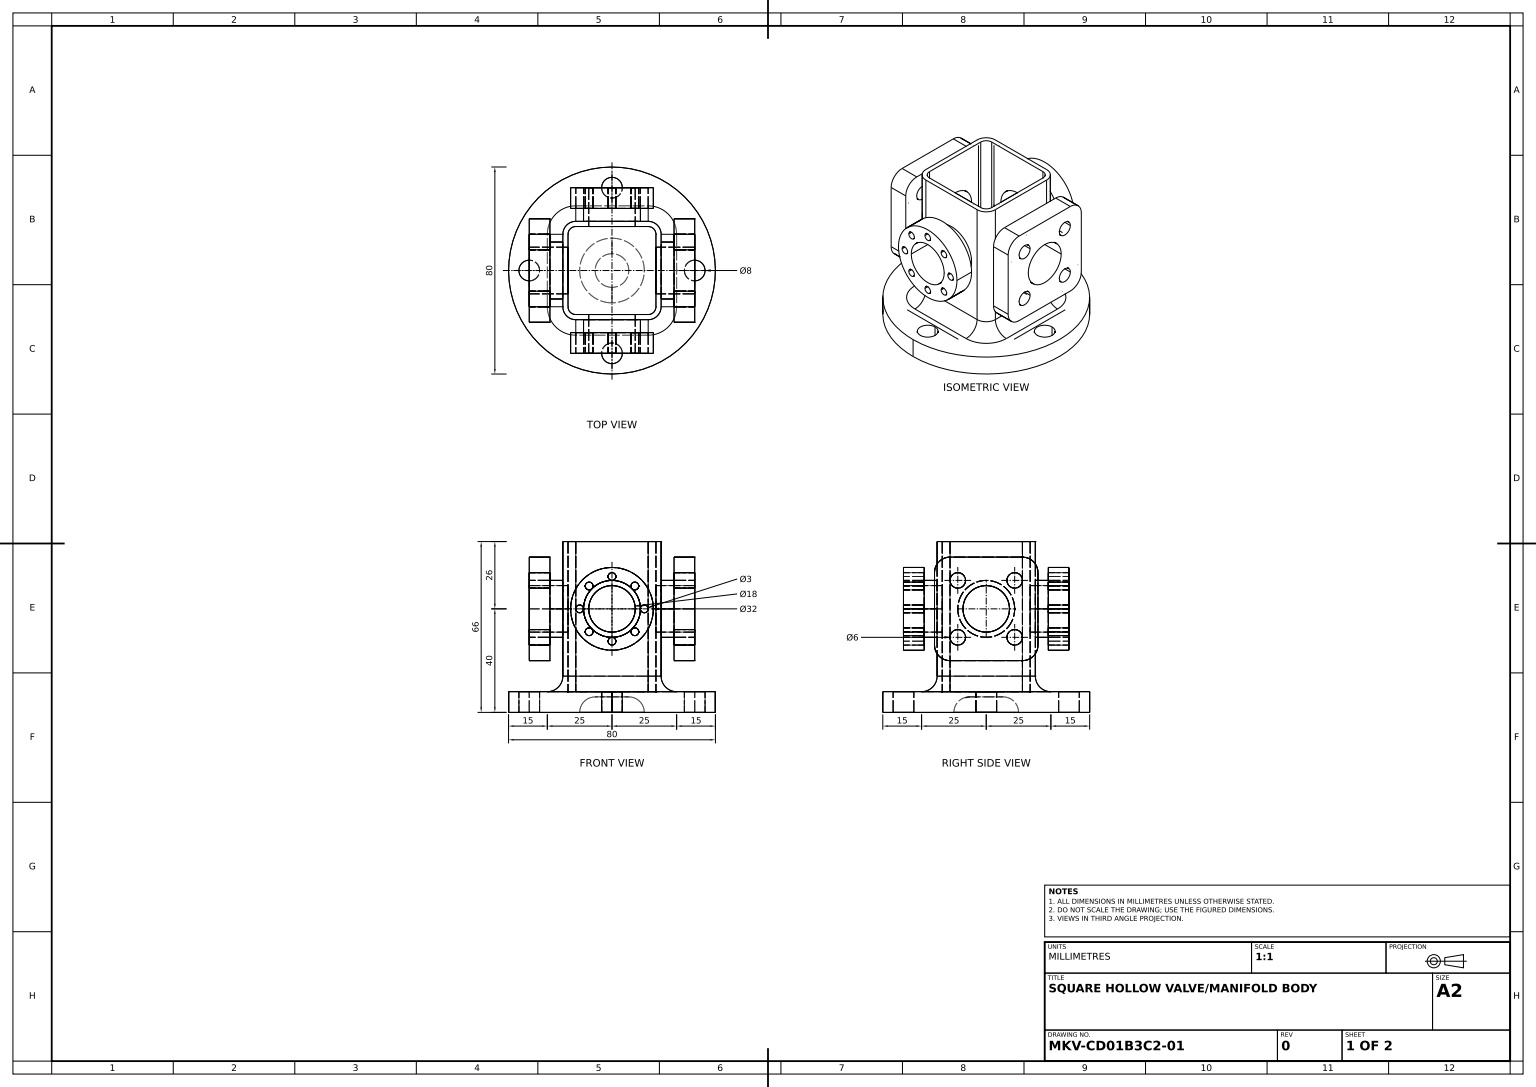
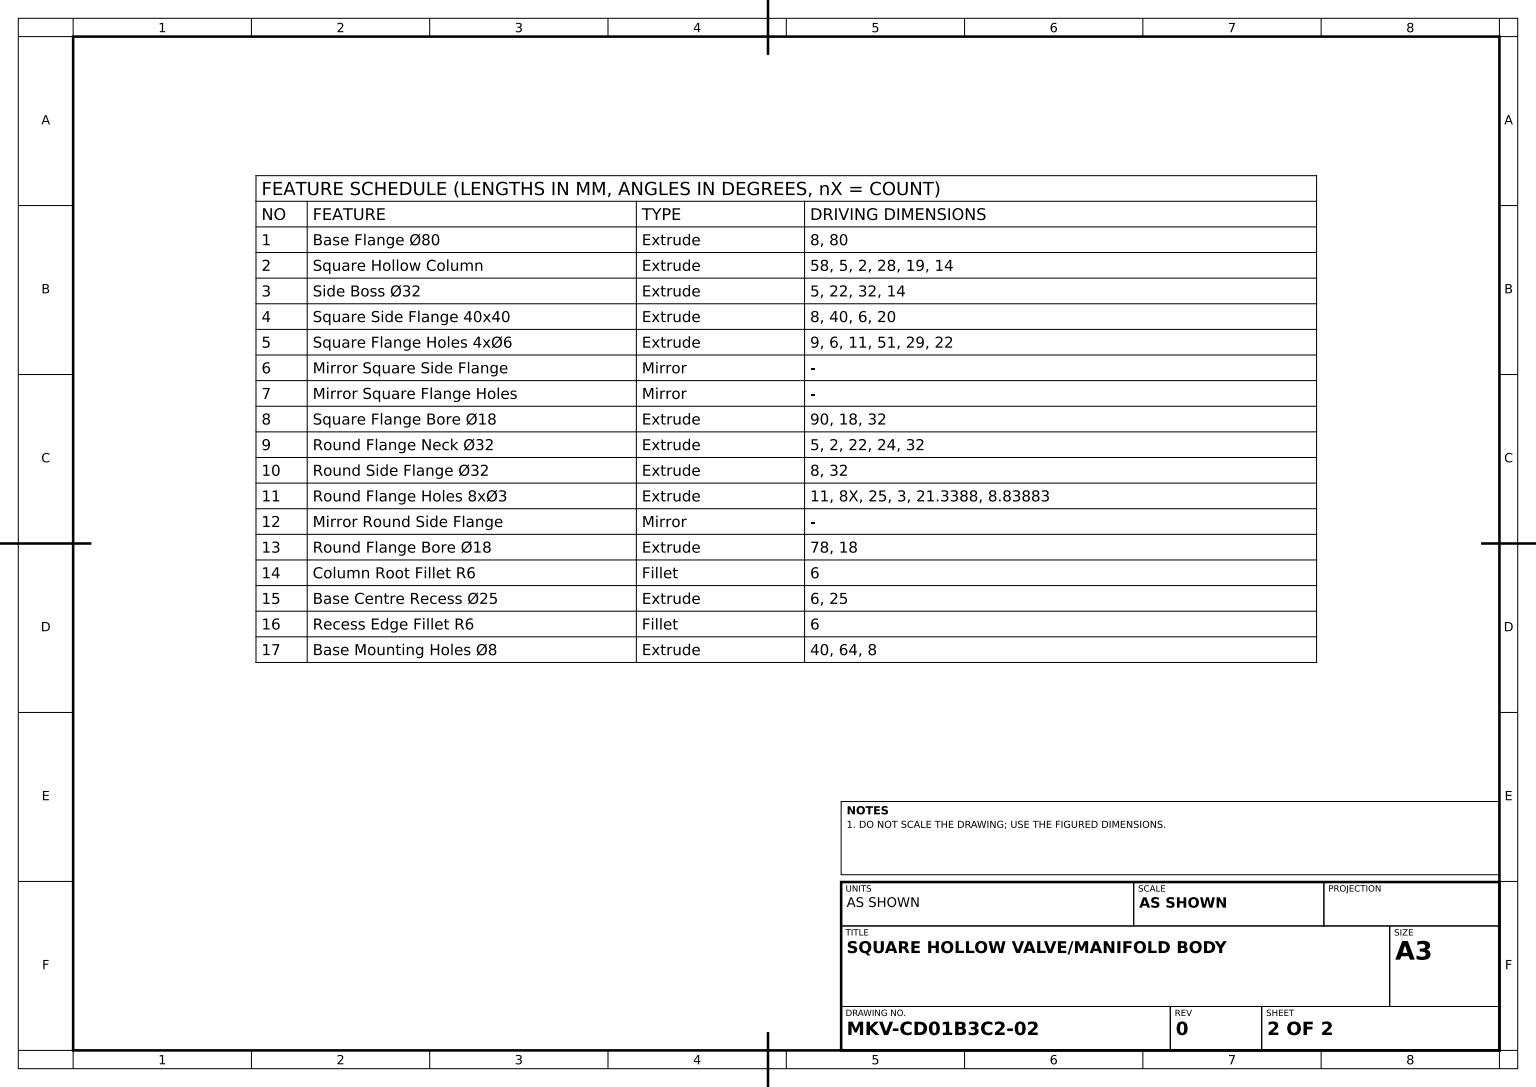
solid
v1 (-24,40,-11)
v2 (-24,40,11)
e1 v1 v2 CIRCLE(AX(P(-24,40,0),D(1,0,0),D(0,0,-1)),11)
v3 (-19,40,11)
e2 v2 v3 LINE
v4 (-19,40,-11)
e3 v4 v3 CIRCLE(AX(P(-19,40,0),D(1,0,0),D(0,0,-1)),11)
e4 v1 v4 LINE
face CYL(AX(P(-24,40,0),D(1,0,0),D(0,0,-1)),11) [e1 e2 -e3 -e4]
v5 (24,20,14)
v6 (24,20,-14)
e5 v5 v6 LINE
v7 (32,20,-14)
e6 v7 v6 LINE
v8 (32,20,14)
e7 v8 v7 LINE
e8 v8 v5 LINE
face PLANE(AX(P(32,20,14),D(0,1,0),D(0,0,1))) rev [e5 -e6 -e7 e8]
v9 (0,0,36)
v10 (0,8,36)
e9 v9 v10 LINE
v11 (0,8,28)
e10 v10 v11 CIRCLE(AX(P(0,8,32),D(0,1,0),D(0,0,1)),4)
v12 (0,0,28)
e11 v12 v11 LINE
e12 v9 v12 CIRCLE(AX(P(0,0,32),D(0,1,0),D(0,0,1)),4)
face CYL(AX(P(0,-32,32),D(0,1,0),D(0,0,1)),4) rev [e9 e10 -e11 -e12]
v13 (-32,51,14)
v14 (-32,51,8)
e13 v13 v14 CIRCLE(AX(P(-32,51,11),D(1,0,0),D(0,0,1)),3)
v15 (-24,51,14)
e14 v15 v13 LINE
v16 (-24,51,8)
e15 v15 v16 CIRCLE(AX(P(-24,51,11),D(1,0,0),D(0,0,1)),3)
e16 v16 v14 LINE
face CYL(AX(P(-23,51,11),D(-1,0,0),D(0,0,1)),3) rev [-e13 -e14 e15 e16]
v17 (-7.338835,31.161165,-24)
v18 (-7.338835,31.161165,-32)
e17 v17 v18 LINE
v19 (-7.778175,32.221825,-24)
e18 v19 v17 CIRCLE(AX(P(-8.838835,31.161165,-24),D(0,0,-1),D(-1,0,0)),1.5)
v20 (-10.338835,31.161165,-24)
e19 v20 v19 CIRCLE(AX(P(-8.838835,31.161165,-24),D(0,0,-1),D(-1,0,0)),1.5)
v21 (-10.338835,31.161165,-32)
e20 v20 v21 LINE
e21 v21 v18 CIRCLE(AX(P(-8.838835,31.161165,-32),D(0,0,-1),D(-1,0,0)),1.5)
face CYL(AX(P(-8.838835,31.161165,-21),D(0,0,-1),D(-1,0,0)),1.5) rev [-e17 -e18 -e19 e20 e21]
v22 (24,29,14)
v23 (24,29,8)
e22 v22 v23 CIRCLE(AX(P(24,29,11),D(1,0,0),D(0,0,-1)),3)
e23 v23 v22 CIRCLE(AX(P(24,29,11),D(1,0,0),D(0,0,-1)),3)
v24 (24,40,11)
v25 (24,40,-11)
e24 v24 v25 CIRCLE(AX(P(24,40,0),D(1,0,0),D(0,0,-1)),11)
e25 v25 v24 CIRCLE(AX(P(24,40,0),D(1,0,0),D(0,0,-1)),11)
v26 (24,51,14)
v27 (24,51,8)
e26 v26 v27 CIRCLE(AX(P(24,51,11),D(1,0,0),D(0,0,-1)),3)
e27 v27 v26 CIRCLE(AX(P(24,51,11),D(1,0,0),D(0,0,-1)),3)
v28 (24,29,-14)
v29 (24,29,-8)
e28 v28 v29 CIRCLE(AX(P(24,29,-11),D(1,0,0),D(0,0,-1)),3)
e29 v29 v28 CIRCLE(AX(P(24,29,-11),D(1,0,0),D(0,0,-1)),3)
v30 (24,60,14)
v31 (24,54,20)
e30 v30 v31 CIRCLE(AX(P(24,54,14),D(1,0,0),D(0,0,-1)),6)
v32 (24,60,-14)
e31 v32 v30 LINE
v33 (24,54,-20)
e32 v33 v32 CIRCLE(AX(P(24,54,-14),D(1,0,0),D(0,0,-1)),6)
v34 (24,26,-20)
e33 v34 v33 LINE
e34 v6 v34 CIRCLE(AX(P(24,26,-14),D(1,0,0),D(0,0,-1)),6)
v35 (24,26,20)
e35 v35 v5 CIRCLE(AX(P(24,26,14),D(1,0,0),D(0,0,-1)),6)
e36 v31 v35 LINE
v36 (24,51,-8)
v37 (24,51,-14)
e37 v36 v37 CIRCLE(AX(P(24,51,-11),D(1,0,0),D(0,0,-1)),3)
e38 v37 v36 CIRCLE(AX(P(24,51,-11),D(1,0,0),D(0,0,-1)),3)
face PLANE(AX(P(24,54,14),D(1,0,0),D(0,0,-1))) rev [e22 e23] [e24 e25] [e26 e27] [e28 e29] [-e30 -e31 -e32 -e33 -e34 -e5 -e35 -e36] [e37 e38]
v38 (-14,8,-25)
v39 (14,8,-25)
e39 v38 v39 LINE
v40 (-14,14,-19)
e40 v38 v40 CIRCLE(AX(P(-14,14,-25),D(-1,0,0),D(0,0,1)),6)
v41 (14,14,-19)
e41 v41 v40 LINE
e42 v39 v41 CIRCLE(AX(P(14,14,-25),D(-1,0,0),D(0,0,1)),6)
face CYL(AX(P(14,14,-25),D(-1,0,0),D(0,0,1)),6) rev [-e39 e40 -e41 -e42]
v42 (0,0,-28)
v43 (0,8,-28)
e43 v42 v43 LINE
v44 (0,0,-36)
e44 v44 v42 CIRCLE(AX(P(0,0,-32),D(0,1,0),D(0,0,1)),4)
v45 (0,8,-36)
e45 v44 v45 LINE
e46 v45 v43 CIRCLE(AX(P(0,8,-32),D(0,1,0),D(0,0,1)),4)
face CYL(AX(P(0,-32,-32),D(0,1,0),D(0,0,1)),4) rev [-e43 -e44 e45 e46]
v46 (-14,40,24)
v47 (-14,40,32)
e47 v46 v47 LINE
v48 (-11,40,24)
e48 v46 v48 CIRCLE(AX(P(-12.5,40,24),D(0,0,-1),D(1,0,0)),1.5)
v49 (-11,40,32)
e49 v48 v49 LINE
e50 v47 v49 CIRCLE(AX(P(-12.5,40,32),D(0,0,-1),D(-1,0,0)),1.5)
face CYL(AX(P(-12.5,40,21),D(0,0,1),D(1,0,0)),1.5) rev [-e47 e48 e49 -e50]
v50 (14,66,19)
v51 (19,66,14)
e51 v50 v51 CIRCLE(AX(P(14,66,14),D(0,1,0),D(0,0,1)),5)
v52 (14,14,19)
e52 v50 v52 LINE
v53 (19,14,14)
e53 v52 v53 CIRCLE(AX(P(14,14,14),D(0,1,0),D(0,0,1)),5)
e54 v51 v53 LINE
face CYL(AX(P(14,66,14),D(0,-1,0),D(0,0,-1)),5) [-e51 e52 e53 -e54]
v54 (1.5,52.5,24)
v55 (1.5,52.5,32)
e55 v54 v55 LINE
v56 (-1.5,52.5,32)
e56 v56 v55 CIRCLE(AX(P(0,52.5,32),D(0,0,-1),D(-1,0,0)),1.5)
v57 (-1.5,52.5,24)
e57 v57 v56 LINE
e58 v57 v54 CIRCLE(AX(P(0,52.5,24),D(0,0,-1),D(1,0,0)),1.5)
face CYL(AX(P(0,52.5,21),D(0,0,1),D(1,0,0)),1.5) rev [e55 -e56 -e57 e58]
v58 (7.778175,47.778175,24)
v59 (11,40,24)
e59 v58 v59 CIRCLE(AX(P(0,40,24),D(0,0,-1),D(-1,0,0)),11)
v60 (11,40,19)
e60 v60 v59 LINE
v61 (-11,40,19)
e61 v60 v61 CIRCLE(AX(P(0,40,19),D(0,0,1),D(-1,0,0)),11)
e62 v61 v48 LINE
v62 (-7.778175,47.778175,24)
e63 v48 v62 CIRCLE(AX(P(0,40,24),D(0,0,-1),D(-1,0,0)),11)
v63 (0,51,24)
e64 v62 v63 CIRCLE(AX(P(0,40,24),D(0,0,-1),D(-1,0,0)),11)
e65 v63 v58 CIRCLE(AX(P(0,40,24),D(0,0,-1),D(-1,0,0)),11)
face CYL(AX(P(0,40,17),D(0,0,1),D(1,0,0)),11) [e59 -e60 e61 e62 e63 e64 e65]
e66 v11 v10 CIRCLE(AX(P(0,8,32),D(0,1,0),D(0,0,1)),4)
e67 v12 v9 CIRCLE(AX(P(0,0,32),D(0,1,0),D(0,0,1)),4)
face CYL(AX(P(0,-32,32),D(0,1,0),D(0,0,1)),4) rev [e66 -e9 -e67 e11]
e68 v43 v45 CIRCLE(AX(P(0,8,-32),D(0,1,0),D(0,0,1)),4)
e69 v42 v44 CIRCLE(AX(P(0,0,-32),D(0,1,0),D(0,0,1)),4)
face CYL(AX(P(0,-32,-32),D(0,1,0),D(0,0,1)),4) rev [e68 -e45 -e69 e43]
v64 (-32,20,-14)
v65 (-32,26,-20)
e70 v64 v65 CIRCLE(AX(P(-32,26,-14),D(1,0,0),D(0,0,-1)),6)
v66 (-24,26,-20)
e71 v65 v66 LINE
v67 (-24,20,-14)
e72 v67 v66 CIRCLE(AX(P(-24,26,-14),D(1,0,0),D(0,0,-1)),6)
e73 v64 v67 LINE
face CYL(AX(P(-32,26,-14),D(1,0,0),D(0,0,-1)),6) [e70 e71 -e72 -e73]
v68 (9,40,-32)
v69 (9,40,-17)
e74 v68 v69 LINE
v70 (-9,40,-17)
e75 v69 v70 CIRCLE(AX(P(0,40,-17),D(0,0,1),D(1,0,0)),9)
v71 (-9,40,-32)
e76 v71 v70 LINE
e77 v71 v68 CIRCLE(AX(P(0,40,-32),D(0,0,-1),D(-1,0,0)),9)
face CYL(AX(P(0,40,-46),D(0,0,1),D(1,0,0)),9) rev [e74 e75 -e76 e77]
v72 (-32,54,-20)
v73 (-32,60,-14)
e78 v72 v73 CIRCLE(AX(P(-32,54,-14),D(1,0,0),D(0,0,-1)),6)
v74 (-24,60,-14)
e79 v73 v74 LINE
v75 (-24,54,-20)
e80 v75 v74 CIRCLE(AX(P(-24,54,-14),D(1,0,0),D(0,0,-1)),6)
e81 v72 v75 LINE
face CYL(AX(P(-32,54,-14),D(1,0,0),D(0,0,-1)),6) [e78 e79 -e80 -e81]
v76 (-17,66,14)
v77 (-17,8,14)
e82 v76 v77 LINE
v78 (-14,66,17)
e83 v76 v78 CIRCLE(AX(P(-14,66,14),D(0,1,0),D(0,0,1)),3)
v79 (-14,8,17)
e84 v78 v79 LINE
e85 v77 v79 CIRCLE(AX(P(-14,8,14),D(0,1,0),D(0,0,1)),3)
face CYL(AX(P(-14,66,14),D(0,-1,0),D(0,0,-1)),3) rev [-e82 e83 e84 -e85]
e86 v49 v47 CIRCLE(AX(P(-12.5,40,32),D(0,0,-1),D(-1,0,0)),1.5)
e87 v48 v46 CIRCLE(AX(P(-12.5,40,24),D(0,0,-1),D(1,0,0)),1.5)
face CYL(AX(P(-12.5,40,21),D(0,0,1),D(1,0,0)),1.5) rev [-e86 -e49 e87 e47]
v80 (14,8,25)
v81 (-14,8,25)
e88 v80 v81 LINE
e89 v52 v80 CIRCLE(AX(P(14,14,25),D(-1,0,0),D(0,-1,0)),6)
v82 (-14,14,19)
e90 v82 v52 LINE
e91 v82 v81 CIRCLE(AX(P(-14,14,25),D(-1,0,0),D(0,0,1)),6)
face CYL(AX(P(-14,14,25),D(1,0,0),D(0,0,-1)),6) rev [-e88 -e89 -e90 e91]
v83 (7.338835,48.838835,-24)
v84 (7.338835,48.838835,-32)
e92 v83 v84 LINE
v85 (7.778175,47.778175,-24)
e93 v85 v83 CIRCLE(AX(P(8.838835,48.838835,-24),D(0,0,-1),D(-1,0,0)),1.5)
v86 (10.338835,48.838835,-24)
e94 v86 v85 CIRCLE(AX(P(8.838835,48.838835,-24),D(0,0,-1),D(-1,0,0)),1.5)
v87 (10.338835,48.838835,-32)
e95 v86 v87 LINE
e96 v87 v84 CIRCLE(AX(P(8.838835,48.838835,-32),D(0,0,-1),D(-1,0,0)),1.5)
face CYL(AX(P(8.838835,48.838835,-21),D(0,0,-1),D(-1,0,0)),1.5) rev [-e92 -e93 -e94 e95 e96]
v88 (14,40,24)
v89 (14,40,32)
e97 v88 v89 LINE
v90 (11,40,32)
e98 v90 v89 CIRCLE(AX(P(12.5,40,32),D(0,0,-1),D(-1,0,0)),1.5)
e99 v59 v90 LINE
e100 v59 v88 CIRCLE(AX(P(12.5,40,24),D(0,0,-1),D(1,0,0)),1.5)
face CYL(AX(P(12.5,40,21),D(0,0,1),D(1,0,0)),1.5) rev [e97 -e98 -e99 e100]
v91 (-24,60,14)
e101 v74 v91 LINE
v92 (-32,60,14)
e102 v73 v92 LINE
e103 v92 v91 LINE
face PLANE(AX(P(-32,60,-14),D(0,1,0),D(0,0,1))) [-e101 -e79 e102 e103]
v93 (25,8,14)
e104 v93 v80 CIRCLE(AX(P(14,8,14),D(0,-1,0),D(0,0,1)),11)
e105 v93 v53 CIRCLE(AX(P(25,14,14),D(0,0,-1),D(-1,0,0)),6)
face TORUS(AX(P(14,14,14),D(0,1,0),D(0,0,1)),11,6) rev [-e53 e89 -e104 e105]
v94 (32,29,14)
e106 v22 v94 LINE
v95 (32,29,8)
e107 v94 v95 CIRCLE(AX(P(32,29,11),D(1,0,0),D(0,0,-1)),3)
e108 v23 v95 LINE
face CYL(AX(P(23,29,11),D(1,0,0),D(0,0,-1)),3) rev [e106 e107 -e108 -e22]
v96 (-24,29,8)
v97 (-24,29,14)
e109 v96 v97 CIRCLE(AX(P(-24,29,11),D(1,0,0),D(0,0,1)),3)
v98 (-32,29,14)
e110 v97 v98 LINE
v99 (-32,29,8)
e111 v99 v98 CIRCLE(AX(P(-32,29,11),D(1,0,0),D(0,0,-1)),3)
e112 v96 v99 LINE
face CYL(AX(P(-23,29,11),D(-1,0,0),D(0,0,1)),3) rev [e109 e110 -e111 -e112]
v100 (0,0,12.5)
v101 (0,0,-12.5)
e113 v100 v101 CIRCLE(AX(P(0,0,0),D(0,-1,0),D(0,0,-1)),12.5)
e114 v101 v100 CIRCLE(AX(P(0,0,0),D(0,-1,0),D(0,0,-1)),12.5)
v102 (0,0,40)
v103 (0,0,-40)
e115 v102 v103 CIRCLE(AX(P(0,0,0),D(0,1,0),D(0,0,1)),40)
e116 v103 v102 CIRCLE(AX(P(0,0,0),D(0,1,0),D(0,0,1)),40)
v104 (-32,0,4)
v105 (-32,0,-4)
e117 v104 v105 CIRCLE(AX(P(-32,0,0),D(0,1,0),D(0,0,1)),4)
e118 v105 v104 CIRCLE(AX(P(-32,0,0),D(0,1,0),D(0,0,1)),4)
v106 (32,0,4)
v107 (32,0,-4)
e119 v106 v107 CIRCLE(AX(P(32,0,0),D(0,1,0),D(0,0,1)),4)
e120 v107 v106 CIRCLE(AX(P(32,0,0),D(0,1,0),D(0,0,1)),4)
face PLANE(AX(P(0,0,0),D(0,1,0),D(0,0,1))) rev [-e113 -e114] [-e115 -e116] [e44 e69] [e117 e118] [e12 e67] [e119 e120]
v108 (-32,54,20)
e121 v92 v108 CIRCLE(AX(P(-32,54,14),D(1,0,0),D(0,0,-1)),6)
v109 (-24,54,20)
e122 v108 v109 LINE
e123 v91 v109 CIRCLE(AX(P(-24,54,14),D(1,0,0),D(0,0,-1)),6)
face CYL(AX(P(-32,54,14),D(1,0,0),D(0,0,-1)),6) [e121 e122 -e123 -e103]
v110 (-7.338835,48.838835,24)
v111 (-7.338835,48.838835,32)
e124 v110 v111 LINE
v112 (-10.338835,48.838835,32)
e125 v112 v111 CIRCLE(AX(P(-8.838835,48.838835,32),D(0,0,-1),D(-1,0,0)),1.5)
v113 (-10.338835,48.838835,24)
e126 v113 v112 LINE
e127 v113 v110 CIRCLE(AX(P(-8.838835,48.838835,24),D(0,0,-1),D(1,0,0)),1.5)
face CYL(AX(P(-8.838835,48.838835,21),D(0,0,1),D(1,0,0)),1.5) rev [e124 -e125 -e126 e127]
e128 v68 v71 CIRCLE(AX(P(0,40,-32),D(0,0,-1),D(-1,0,0)),9)
e129 v70 v69 CIRCLE(AX(P(0,40,-17),D(0,0,1),D(1,0,0)),9)
face CYL(AX(P(0,40,-46),D(0,0,1),D(1,0,0)),9) rev [e128 e76 e129 -e74]
v114 (32,54,20)
v115 (32,26,20)
e130 v114 v115 LINE
e131 v114 v31 LINE
e132 v115 v35 LINE
face PLANE(AX(P(32,54,20),D(0,0,-1),D(0,1,0))) rev [-e130 e131 e36 -e132]
v116 (-32,8,-4)
e133 v105 v116 LINE
v117 (-32,8,4)
e134 v104 v117 LINE
e135 v117 v116 CIRCLE(AX(P(-32,8,0),D(0,1,0),D(0,0,1)),4)
face CYL(AX(P(-32,-32,0),D(0,1,0),D(0,0,1)),4) rev [-e133 -e117 e134 e135]
v118 (32,26,-20)
e136 v118 v34 LINE
e137 v7 v118 CIRCLE(AX(P(32,26,-14),D(1,0,0),D(0,0,-1)),6)
face CYL(AX(P(32,26,-14),D(-1,0,0),D(0,0,1)),6) [e6 e34 -e136 -e137]
v119 (-10.338835,31.161165,24)
v120 (-10.338835,31.161165,32)
e138 v119 v120 LINE
v121 (-7.338835,31.161165,32)
e139 v121 v120 CIRCLE(AX(P(-8.838835,31.161165,32),D(0,0,-1),D(-1,0,0)),1.5)
v122 (-7.338835,31.161165,24)
e140 v122 v121 LINE
e141 v122 v119 CIRCLE(AX(P(-8.838835,31.161165,24),D(0,0,-1),D(1,0,0)),1.5)
face CYL(AX(P(-8.838835,31.161165,21),D(0,0,1),D(1,0,0)),1.5) rev [e138 -e139 -e140 e141]
v123 (-11,40,-19)
v124 (-11,40,-24)
e142 v123 v124 LINE
e143 v19 v124 CIRCLE(AX(P(0,40,-24),D(0,0,-1),D(-1,0,0)),11)
v125 (0,29,-24)
e144 v125 v19 CIRCLE(AX(P(0,40,-24),D(0,0,-1),D(-1,0,0)),11)
v126 (7.778175,32.221825,-24)
e145 v126 v125 CIRCLE(AX(P(0,40,-24),D(0,0,-1),D(-1,0,0)),11)
v127 (11,40,-24)
e146 v127 v126 CIRCLE(AX(P(0,40,-24),D(0,0,-1),D(-1,0,0)),11)
v128 (11,40,-19)
e147 v128 v127 LINE
e148 v123 v128 CIRCLE(AX(P(0,40,-19),D(0,0,1),D(1,0,0)),11)
face CYL(AX(P(0,40,-17),D(0,0,-1),D(-1,0,0)),11) [e142 -e143 -e144 -e145 -e146 -e147 -e148]
v129 (32,60,14)
e149 v129 v114 CIRCLE(AX(P(32,54,14),D(1,0,0),D(0,0,-1)),6)
e150 v129 v30 LINE
face CYL(AX(P(32,54,14),D(-1,0,0),D(0,0,1)),6) [-e131 -e149 e150 e30]
v130 (0,8,40)
v131 (0,8,-40)
e151 v130 v131 CIRCLE(AX(P(0,8,0),D(0,1,0),D(0,0,1)),40)
e152 v131 v130 CIRCLE(AX(P(0,8,0),D(0,1,0),D(0,0,1)),40)
v132 (-25,8,14)
e153 v81 v132 CIRCLE(AX(P(-14,8,14),D(0,-1,0),D(0,0,1)),11)
v133 (-25,8,-14)
e154 v132 v133 LINE
e155 v133 v38 CIRCLE(AX(P(-14,8,-14),D(0,-1,0),D(0,0,1)),11)
v134 (25,8,-14)
e156 v39 v134 CIRCLE(AX(P(14,8,-14),D(0,-1,0),D(0,0,1)),11)
e157 v134 v93 LINE
e158 v116 v117 CIRCLE(AX(P(-32,8,0),D(0,1,0),D(0,0,1)),4)
v135 (32,8,-4)
v136 (32,8,4)
e159 v135 v136 CIRCLE(AX(P(32,8,0),D(0,1,0),D(0,0,1)),4)
e160 v136 v135 CIRCLE(AX(P(32,8,0),D(0,1,0),D(0,0,1)),4)
face PLANE(AX(P(0,8,0),D(0,1,0),D(0,0,1))) [e151 e152] [-e66 -e10] [e104 e88 e153 e154 e155 e39 e156 e157] [-e68 -e46] [-e135 -e158] [-e159 -e160]
v137 (32,29,-14)
e161 v28 v137 LINE
v138 (32,29,-8)
e162 v29 v138 LINE
e163 v138 v137 CIRCLE(AX(P(32,29,-11),D(1,0,0),D(0,0,1)),3)
face CYL(AX(P(23,29,-11),D(1,0,0),D(0,0,-1)),3) rev [-e161 -e29 e162 e163]
face CYL(AX(P(-32,-32,0),D(0,1,0),D(0,0,1)),4) rev [e158 -e134 -e118 e133]
v139 (0,51,-24)
v140 (-1.5,52.5,-24)
e164 v139 v140 CIRCLE(AX(P(0,52.5,-24),D(0,0,-1),D(-1,0,0)),1.5)
v141 (1.5,52.5,-24)
e165 v141 v139 CIRCLE(AX(P(0,52.5,-24),D(0,0,-1),D(-1,0,0)),1.5)
v142 (1.5,52.5,-32)
e166 v141 v142 LINE
v143 (-1.5,52.5,-32)
e167 v142 v143 CIRCLE(AX(P(0,52.5,-32),D(0,0,-1),D(-1,0,0)),1.5)
e168 v140 v143 LINE
face CYL(AX(P(0,52.5,-21),D(0,0,-1),D(-1,0,0)),1.5) rev [-e164 -e165 e166 e167 -e168]
v144 (-24,20,14)
e169 v144 v67 LINE
v145 (-32,20,14)
e170 v145 v144 LINE
e171 v145 v64 LINE
face PLANE(AX(P(-32,20,14),D(0,-1,0),D(0,0,-1))) [e73 -e169 -e170 e171]
v146 (-14,40,-24)
e172 v124 v146 CIRCLE(AX(P(-12.5,40,-24),D(0,0,-1),D(-1,0,0)),1.5)
v147 (-11,40,-32)
e173 v124 v147 LINE
v148 (-14,40,-32)
e174 v147 v148 CIRCLE(AX(P(-12.5,40,-32),D(0,0,-1),D(-1,0,0)),1.5)
e175 v146 v148 LINE
face CYL(AX(P(-12.5,40,-21),D(0,0,-1),D(-1,0,0)),1.5) rev [-e172 e173 e174 -e175]
v149 (32,40,-9)
v150 (17,40,-9)
e176 v149 v150 LINE
v151 (17,40,9)
e177 v150 v151 CIRCLE(AX(P(17,40,0),D(-1,0,0),D(0,0,1)),9)
v152 (32,40,9)
e178 v152 v151 LINE
e179 v152 v149 CIRCLE(AX(P(32,40,0),D(1,0,0),D(0,0,-1)),9)
face CYL(AX(P(58,40,0),D(-1,0,0),D(0,0,1)),9) rev [e176 e177 -e178 e179]
e180 v14 v13 CIRCLE(AX(P(-32,51,11),D(1,0,0),D(0,0,1)),3)
e181 v16 v15 CIRCLE(AX(P(-24,51,11),D(1,0,0),D(0,0,1)),3)
face CYL(AX(P(-23,51,11),D(-1,0,0),D(0,0,1)),3) rev [-e180 -e16 e181 e14]
v153 (32,51,-8)
e182 v36 v153 LINE
v154 (32,51,-14)
e183 v153 v154 CIRCLE(AX(P(32,51,-11),D(1,0,0),D(0,0,-1)),3)
e184 v37 v154 LINE
face CYL(AX(P(23,51,-11),D(1,0,0),D(0,0,-1)),3) rev [e182 e183 -e184 -e37]
v155 (-17,40,-9)
v156 (-17,40,9)
e185 v155 v156 CIRCLE(AX(P(-17,40,0),D(1,0,0),D(0,0,-1)),9)
v157 (-32,40,9)
e186 v156 v157 LINE
v158 (-32,40,-9)
e187 v157 v158 CIRCLE(AX(P(-32,40,0),D(-1,0,0),D(0,0,1)),9)
e188 v155 v158 LINE
face CYL(AX(P(58,40,0),D(-1,0,0),D(0,0,1)),9) rev [e185 e186 e187 -e188]
v159 (-16,40,32)
v160 (-16,40,24)
e189 v159 v160 LINE
v161 (16,40,24)
e190 v161 v160 CIRCLE(AX(P(0,40,24),D(0,0,-1),D(-1,0,0)),16)
v162 (16,40,32)
e191 v162 v161 LINE
e192 v162 v159 CIRCLE(AX(P(0,40,32),D(0,0,-1),D(-1,0,0)),16)
face CYL(AX(P(0,40,32),D(0,0,-1),D(-1,0,0)),16) [e189 -e190 -e191 e192]
e193 v120 v121 CIRCLE(AX(P(-8.838835,31.161165,32),D(0,0,-1),D(-1,0,0)),1.5)
v163 (-7.778175,32.221825,24)
e194 v119 v163 CIRCLE(AX(P(-8.838835,31.161165,24),D(0,0,-1),D(1,0,0)),1.5)
e195 v163 v122 CIRCLE(AX(P(-8.838835,31.161165,24),D(0,0,-1),D(1,0,0)),1.5)
face CYL(AX(P(-8.838835,31.161165,21),D(0,0,1),D(1,0,0)),1.5) rev [-e193 -e138 e194 e195 e140]
v164 (1.5,27.5,32)
v165 (-1.5,27.5,32)
e196 v164 v165 CIRCLE(AX(P(0,27.5,32),D(0,0,-1),D(-1,0,0)),1.5)
v166 (1.5,27.5,24)
e197 v166 v164 LINE
v167 (-1.5,27.5,24)
e198 v166 v167 CIRCLE(AX(P(0,27.5,24),D(0,0,-1),D(1,0,0)),1.5)
e199 v167 v165 LINE
face CYL(AX(P(0,27.5,21),D(0,0,1),D(1,0,0)),1.5) rev [-e196 -e197 e198 e199]
e200 v151 v150 CIRCLE(AX(P(17,40,0),D(-1,0,0),D(0,0,1)),9)
e201 v149 v152 CIRCLE(AX(P(32,40,0),D(1,0,0),D(0,0,-1)),9)
face CYL(AX(P(58,40,0),D(-1,0,0),D(0,0,1)),9) rev [e200 -e176 e201 e178]
e202 v137 v138 CIRCLE(AX(P(32,29,-11),D(1,0,0),D(0,0,1)),3)
face CYL(AX(P(23,29,-11),D(1,0,0),D(0,0,-1)),3) rev [-e28 e161 e202 -e162]
e203 v61 v60 CIRCLE(AX(P(0,40,19),D(0,0,1),D(-1,0,0)),11)
v168 (-14,66,19)
e204 v168 v50 LINE
e205 v168 v82 LINE
face PLANE(AX(P(-14,66,19),D(0,0,-1),D(-1,0,0))) rev [-e203 -e61] [-e52 -e204 e205 e90]
v169 (16,40,-24)
v170 (-16,40,-24)
e206 v169 v170 CIRCLE(AX(P(0,40,-24),D(0,0,-1),D(-1,0,0)),16)
v171 (-16,40,-32)
e207 v171 v170 LINE
v172 (16,40,-32)
e208 v172 v171 CIRCLE(AX(P(0,40,-32),D(0,0,-1),D(-1,0,0)),16)
e209 v172 v169 LINE
face CYL(AX(P(0,40,-32),D(0,0,1),D(1,0,0)),16) [e206 -e207 -e208 e209]
v173 (19,40,11)
v174 (19,40,-11)
e210 v173 v174 CIRCLE(AX(P(19,40,0),D(1,0,0),D(0,0,1)),11)
e211 v174 v173 CIRCLE(AX(P(19,40,0),D(1,0,0),D(0,0,1)),11)
v175 (19,14,-14)
e212 v53 v175 LINE
v176 (19,66,-14)
e213 v176 v175 LINE
e214 v51 v176 LINE
face PLANE(AX(P(19,66,0),D(-1,0,0),D(0,0,1))) rev [-e210 -e211] [e54 e212 -e213 -e214]
e215 v55 v56 CIRCLE(AX(P(0,52.5,32),D(0,0,-1),D(-1,0,0)),1.5)
e216 v54 v63 CIRCLE(AX(P(0,52.5,24),D(0,0,-1),D(1,0,0)),1.5)
e217 v63 v57 CIRCLE(AX(P(0,52.5,24),D(0,0,-1),D(1,0,0)),1.5)
face CYL(AX(P(0,52.5,21),D(0,0,1),D(1,0,0)),1.5) rev [-e215 -e55 e216 e217 e57]
v177 (14,40,-24)
v178 (14,40,-32)
e218 v177 v178 LINE
e219 v127 v177 CIRCLE(AX(P(12.5,40,-24),D(0,0,-1),D(-1,0,0)),1.5)
v179 (11,40,-32)
e220 v127 v179 LINE
e221 v179 v178 CIRCLE(AX(P(12.5,40,-32),D(0,0,-1),D(-1,0,0)),1.5)
face CYL(AX(P(12.5,40,-21),D(0,0,-1),D(-1,0,0)),1.5) rev [-e218 -e219 e220 e221]
v180 (-24,51,-14)
v181 (-24,51,-8)
e222 v180 v181 CIRCLE(AX(P(-24,51,-11),D(1,0,0),D(0,0,1)),3)
v182 (-32,51,-8)
e223 v181 v182 LINE
v183 (-32,51,-14)
e224 v183 v182 CIRCLE(AX(P(-32,51,-11),D(1,0,0),D(0,0,-1)),3)
e225 v180 v183 LINE
face CYL(AX(P(-23,51,-11),D(-1,0,0),D(0,0,1)),3) rev [e222 e223 -e224 -e225]
v184 (9,40,17)
v185 (-9,40,17)
e226 v184 v185 CIRCLE(AX(P(0,40,17),D(0,0,-1),D(-1,0,0)),9)
v186 (-9,40,32)
e227 v185 v186 LINE
v187 (9,40,32)
e228 v186 v187 CIRCLE(AX(P(0,40,32),D(0,0,1),D(1,0,0)),9)
e229 v184 v187 LINE
face CYL(AX(P(0,40,-46),D(0,0,1),D(1,0,0)),9) rev [e226 e227 e228 -e229]
e230 v98 v99 CIRCLE(AX(P(-32,29,11),D(1,0,0),D(0,0,-1)),3)
v188 (-32,26,20)
e231 v188 v145 CIRCLE(AX(P(-32,26,14),D(1,0,0),D(0,0,-1)),6)
e232 v108 v188 LINE
e233 v65 v72 LINE
v189 (-32,29,-14)
v190 (-32,29,-8)
e234 v189 v190 CIRCLE(AX(P(-32,29,-11),D(1,0,0),D(0,0,1)),3)
e235 v190 v189 CIRCLE(AX(P(-32,29,-11),D(1,0,0),D(0,0,1)),3)
e236 v158 v157 CIRCLE(AX(P(-32,40,0),D(-1,0,0),D(0,0,1)),9)
e237 v182 v183 CIRCLE(AX(P(-32,51,-11),D(1,0,0),D(0,0,-1)),3)
face PLANE(AX(P(-32,54,14),D(-1,0,0),D(0,0,-1))) [e230 e111] [e13 e180] [-e171 -e231 -e232 -e121 -e102 -e78 -e233 -e70] [e234 e235] [-e187 -e236] [e224 e237]
v191 (32,51,8)
e238 v27 v191 LINE
v192 (32,51,14)
e239 v26 v192 LINE
e240 v192 v191 CIRCLE(AX(P(32,51,11),D(1,0,0),D(0,0,1)),3)
face CYL(AX(P(23,51,11),D(1,0,0),D(0,0,-1)),3) rev [-e238 -e26 e239 e240]
e241 v130 v102 LINE
e242 v131 v103 LINE
face CYL(AX(P(0,8,0),D(0,-1,0),D(0,0,-1)),40) [e116 -e241 -e152 e242]
v193 (0,6,-6.5)
e243 v193 v101 CIRCLE(AX(P(0,0,-6.5),D(-1,0,0),D(0,0,1)),6)
v194 (0,6,6.5)
e244 v194 v193 CIRCLE(AX(P(0,6,0),D(0,-1,0),D(0,0,-1)),6.5)
e245 v194 v100 CIRCLE(AX(P(0,0,6.5),D(1,0,0),D(0,0,-1)),6)
face TORUS(AX(P(0,0,0),D(0,-1,0),D(0,0,-1)),6.5,6) rev [e113 -e243 -e244 e245]
v195 (32,60,-14)
e246 v195 v32 LINE
v196 (32,54,-20)
e247 v196 v195 CIRCLE(AX(P(32,54,-14),D(1,0,0),D(0,0,-1)),6)
e248 v196 v33 LINE
face CYL(AX(P(32,54,-14),D(-1,0,0),D(0,0,1)),6) [-e246 -e247 e248 e32]
e249 v181 v180 CIRCLE(AX(P(-24,51,-11),D(1,0,0),D(0,0,1)),3)
face CYL(AX(P(-23,51,-11),D(-1,0,0),D(0,0,1)),3) rev [e225 -e237 -e223 e249]
e250 v2 v1 CIRCLE(AX(P(-24,40,0),D(1,0,0),D(0,0,-1)),11)
e251 v3 v4 CIRCLE(AX(P(-19,40,0),D(1,0,0),D(0,0,-1)),11)
face CYL(AX(P(-24,40,0),D(1,0,0),D(0,0,-1)),11) [e250 e4 -e251 -e2]
v197 (-1.5,27.5,-24)
e252 v197 v125 CIRCLE(AX(P(0,27.5,-24),D(0,0,-1),D(-1,0,0)),1.5)
v198 (-1.5,27.5,-32)
e253 v197 v198 LINE
v199 (1.5,27.5,-32)
e254 v198 v199 CIRCLE(AX(P(0,27.5,-32),D(0,0,-1),D(-1,0,0)),1.5)
v200 (1.5,27.5,-24)
e255 v200 v199 LINE
e256 v125 v200 CIRCLE(AX(P(0,27.5,-24),D(0,0,-1),D(-1,0,0)),1.5)
face CYL(AX(P(0,27.5,-21),D(0,0,-1),D(-1,0,0)),1.5) rev [-e252 e253 e254 -e255 -e256]
e257 v154 v153 CIRCLE(AX(P(32,51,-11),D(1,0,0),D(0,0,-1)),3)
face CYL(AX(P(23,51,-11),D(1,0,0),D(0,0,-1)),3) rev [e184 e257 -e182 -e38]
e258 v128 v123 CIRCLE(AX(P(0,40,-19),D(0,0,1),D(1,0,0)),11)
e259 v85 v127 CIRCLE(AX(P(0,40,-24),D(0,0,-1),D(-1,0,0)),11)
e260 v139 v85 CIRCLE(AX(P(0,40,-24),D(0,0,-1),D(-1,0,0)),11)
v201 (-7.778175,47.778175,-24)
e261 v201 v139 CIRCLE(AX(P(0,40,-24),D(0,0,-1),D(-1,0,0)),11)
e262 v124 v201 CIRCLE(AX(P(0,40,-24),D(0,0,-1),D(-1,0,0)),11)
face CYL(AX(P(0,40,-17),D(0,0,-1),D(-1,0,0)),11) [-e142 -e258 e147 -e259 -e260 -e261 -e262]
e263 v25 v174 LINE
e264 v24 v173 LINE
face CYL(AX(P(24,40,0),D(-1,0,0),D(0,0,1)),11) [-e263 -e24 e264 e210]
e265 v89 v90 CIRCLE(AX(P(12.5,40,32),D(0,0,-1),D(-1,0,0)),1.5)
e266 v88 v59 CIRCLE(AX(P(12.5,40,24),D(0,0,-1),D(1,0,0)),1.5)
face CYL(AX(P(12.5,40,21),D(0,0,1),D(1,0,0)),1.5) rev [-e265 -e97 e266 e99]
e267 v95 v94 CIRCLE(AX(P(32,29,11),D(1,0,0),D(0,0,-1)),3)
face CYL(AX(P(23,29,11),D(1,0,0),D(0,0,-1)),3) rev [-e23 e108 e267 -e106]
v202 (7.778175,32.221825,24)
e268 v59 v202 CIRCLE(AX(P(0,40,24),D(0,0,-1),D(-1,0,0)),11)
v203 (0,29,24)
e269 v202 v203 CIRCLE(AX(P(0,40,24),D(0,0,-1),D(-1,0,0)),11)
e270 v203 v163 CIRCLE(AX(P(0,40,24),D(0,0,-1),D(-1,0,0)),11)
e271 v163 v48 CIRCLE(AX(P(0,40,24),D(0,0,-1),D(-1,0,0)),11)
face CYL(AX(P(0,40,17),D(0,0,1),D(1,0,0)),11) [e268 e269 e270 e271 -e62 e203 e60]
e272 v66 v75 LINE
face PLANE(AX(P(-32,26,-20),D(0,0,-1),D(-1,0,0))) [-e272 -e71 e233 e81]
v204 (14,66,-19)
e273 v204 v41 LINE
e274 v176 v204 CIRCLE(AX(P(14,66,-14),D(0,1,0),D(0,0,1)),5)
e275 v175 v41 CIRCLE(AX(P(14,14,-14),D(0,1,0),D(0,0,1)),5)
face CYL(AX(P(14,66,-14),D(0,-1,0),D(0,0,-1)),5) [-e273 -e274 e213 e275]
e276 v160 v161 CIRCLE(AX(P(0,40,24),D(0,0,-1),D(-1,0,0)),16)
e277 v159 v162 CIRCLE(AX(P(0,40,32),D(0,0,-1),D(-1,0,0)),16)
face CYL(AX(P(0,40,32),D(0,0,-1),D(-1,0,0)),16) [e191 -e276 -e189 e277]
e278 v178 v179 CIRCLE(AX(P(12.5,40,-32),D(0,0,-1),D(-1,0,0)),1.5)
e279 v177 v127 CIRCLE(AX(P(12.5,40,-24),D(0,0,-1),D(-1,0,0)),1.5)
face CYL(AX(P(12.5,40,-21),D(0,0,-1),D(-1,0,0)),1.5) rev [e218 e278 -e220 -e279]
e280 v171 v172 CIRCLE(AX(P(0,40,-32),D(0,0,-1),D(-1,0,0)),16)
e281 v170 v169 CIRCLE(AX(P(0,40,-24),D(0,0,-1),D(-1,0,0)),16)
face CYL(AX(P(0,40,-32),D(0,0,1),D(1,0,0)),16) [-e280 e207 e281 -e209]
e282 v185 v184 CIRCLE(AX(P(0,40,17),D(0,0,-1),D(-1,0,0)),9)
v205 (14,8,17)
e283 v79 v205 LINE
v206 (14,66,17)
e284 v78 v206 LINE
e285 v206 v205 LINE
face PLANE(AX(P(-14,66,17),D(0,0,-1),D(-1,0,0))) [-e226 -e282] [-e283 -e84 e284 e285]
v207 (10.338835,31.161165,-24)
v208 (10.338835,31.161165,-32)
e286 v207 v208 LINE
v209 (7.338835,31.161165,-32)
e287 v208 v209 CIRCLE(AX(P(8.838835,31.161165,-32),D(0,0,-1),D(-1,0,0)),1.5)
v210 (7.338835,31.161165,-24)
e288 v210 v209 LINE
e289 v207 v210 CIRCLE(AX(P(8.838835,31.161165,-24),D(0,0,-1),D(-1,0,0)),1.5)
face CYL(AX(P(8.838835,31.161165,-21),D(0,0,-1),D(-1,0,0)),1.5) rev [e286 e287 -e288 -e289]
e290 v110 v62 CIRCLE(AX(P(-8.838835,48.838835,24),D(0,0,-1),D(1,0,0)),1.5)
e291 v62 v113 CIRCLE(AX(P(-8.838835,48.838835,24),D(0,0,-1),D(1,0,0)),1.5)
e292 v167 v203 CIRCLE(AX(P(0,27.5,24),D(0,0,-1),D(1,0,0)),1.5)
e293 v203 v166 CIRCLE(AX(P(0,27.5,24),D(0,0,-1),D(1,0,0)),1.5)
v211 (7.338835,31.161165,24)
e294 v211 v202 CIRCLE(AX(P(8.838835,31.161165,24),D(0,0,-1),D(1,0,0)),1.5)
v212 (10.338835,31.161165,24)
e295 v212 v211 CIRCLE(AX(P(8.838835,31.161165,24),D(0,0,-1),D(1,0,0)),1.5)
e296 v202 v212 CIRCLE(AX(P(8.838835,31.161165,24),D(0,0,-1),D(1,0,0)),1.5)
v213 (10.338835,48.838835,24)
e297 v213 v58 CIRCLE(AX(P(8.838835,48.838835,24),D(0,0,-1),D(1,0,0)),1.5)
v214 (7.338835,48.838835,24)
e298 v214 v213 CIRCLE(AX(P(8.838835,48.838835,24),D(0,0,-1),D(1,0,0)),1.5)
e299 v58 v214 CIRCLE(AX(P(8.838835,48.838835,24),D(0,0,-1),D(1,0,0)),1.5)
face PLANE(AX(P(0,40,24),D(0,0,1),D(-1,0,0))) rev [e190 e276] [-e290 -e127 -e291 -e63 -e48 -e87 -e271 -e194 -e141 -e195 -e270 -e292 -e198 -e293 -e269 -e294 -e295 -e296 -e268 -e266 -e100 -e59 -e297 -e298 -e299 -e65 -e216 -e58 -e217 -e64]
e300 v118 v196 LINE
face PLANE(AX(P(32,40,-20),D(0,0,1),D(1,0,0))) rev [-e300 e136 e33 -e248]
e301 v195 v129 LINE
e302 v115 v8 CIRCLE(AX(P(32,26,14),D(1,0,0),D(0,0,-1)),6)
e303 v191 v192 CIRCLE(AX(P(32,51,11),D(1,0,0),D(0,0,1)),3)
face PLANE(AX(P(32,54,14),D(1,0,0),D(0,0,-1))) [-e201 -e179] [e7 e137 e300 e247 e301 e149 e130 e302] [-e267 -e107] [-e257 -e183] [-e303 -e240] [-e163 -e202]
v215 (-19,14,-14)
e304 v215 v133 CIRCLE(AX(P(-25,14,-14),D(0,0,-1),D(-1,0,0)),6)
e305 v40 v215 CIRCLE(AX(P(-14,14,-14),D(0,1,0),D(0,0,1)),5)
face TORUS(AX(P(-14,14,-14),D(0,1,0),D(0,0,1)),11,6) rev [-e155 -e304 -e305 -e40]
v216 (10.338835,31.161165,32)
e306 v212 v216 LINE
v217 (7.338835,31.161165,32)
e307 v211 v217 LINE
e308 v216 v217 CIRCLE(AX(P(8.838835,31.161165,32),D(0,0,-1),D(-1,0,0)),1.5)
face CYL(AX(P(8.838835,31.161165,21),D(0,0,1),D(1,0,0)),1.5) rev [-e306 e295 e307 -e308]
v218 (-19,66,-14)
e309 v218 v215 LINE
v219 (-14,66,-19)
e310 v219 v218 CIRCLE(AX(P(-14,66,-14),D(0,1,0),D(0,0,1)),5)
e311 v219 v40 LINE
face CYL(AX(P(-14,66,-14),D(0,-1,0),D(0,0,-1)),5) [-e309 -e310 e311 e305]
v220 (7.338835,48.838835,32)
e312 v214 v220 LINE
v221 (10.338835,48.838835,32)
e313 v213 v221 LINE
e314 v220 v221 CIRCLE(AX(P(8.838835,48.838835,32),D(0,0,-1),D(-1,0,0)),1.5)
face CYL(AX(P(8.838835,48.838835,21),D(0,0,1),D(1,0,0)),1.5) rev [-e312 e298 e313 -e314]
e315 v210 v126 CIRCLE(AX(P(8.838835,31.161165,-24),D(0,0,-1),D(-1,0,0)),1.5)
e316 v200 v197 CIRCLE(AX(P(0,27.5,-24),D(0,0,-1),D(-1,0,0)),1.5)
e317 v17 v20 CIRCLE(AX(P(-8.838835,31.161165,-24),D(0,0,-1),D(-1,0,0)),1.5)
e318 v146 v124 CIRCLE(AX(P(-12.5,40,-24),D(0,0,-1),D(-1,0,0)),1.5)
v222 (-10.338835,48.838835,-24)
e319 v201 v222 CIRCLE(AX(P(-8.838835,48.838835,-24),D(0,0,-1),D(-1,0,0)),1.5)
v223 (-7.338835,48.838835,-24)
e320 v222 v223 CIRCLE(AX(P(-8.838835,48.838835,-24),D(0,0,-1),D(-1,0,0)),1.5)
e321 v223 v201 CIRCLE(AX(P(-8.838835,48.838835,-24),D(0,0,-1),D(-1,0,0)),1.5)
e322 v140 v141 CIRCLE(AX(P(0,52.5,-24),D(0,0,-1),D(-1,0,0)),1.5)
e323 v83 v86 CIRCLE(AX(P(8.838835,48.838835,-24),D(0,0,-1),D(-1,0,0)),1.5)
e324 v126 v207 CIRCLE(AX(P(8.838835,31.161165,-24),D(0,0,-1),D(-1,0,0)),1.5)
face PLANE(AX(P(0,40,-24),D(0,0,-1),D(-1,0,0))) rev [e315 e145 e256 e316 e252 e144 e18 e317 e19 e143 e172 e318 e262 e319 e320 e321 e261 e164 e322 e165 e260 e93 e323 e94 e259 e219 e279 e146 e324 e289] [-e206 -e281]
v224 (14,66,-17)
v225 (14,8,-17)
e325 v224 v225 LINE
v226 (17,8,-14)
e326 v226 v225 CIRCLE(AX(P(14,8,-14),D(0,1,0),D(0,0,1)),3)
v227 (17,66,-14)
e327 v227 v226 LINE
e328 v227 v224 CIRCLE(AX(P(14,66,-14),D(0,1,0),D(0,0,1)),3)
face CYL(AX(P(14,66,-14),D(0,-1,0),D(0,0,-1)),3) rev [e325 -e326 -e327 e328]
e329 v134 v175 CIRCLE(AX(P(25,14,-14),D(0,0,-1),D(-1,0,0)),6)
face TORUS(AX(P(14,14,-14),D(0,1,0),D(0,0,1)),11,6) rev [-e156 e42 -e275 -e329]
e330 v18 v21 CIRCLE(AX(P(-8.838835,31.161165,-32),D(0,0,-1),D(-1,0,0)),1.5)
face CYL(AX(P(-8.838835,31.161165,-21),D(0,0,-1),D(-1,0,0)),1.5) rev [e17 e330 -e20 -e317]
v228 (-19,14,14)
e331 v228 v82 CIRCLE(AX(P(-14,14,14),D(0,1,0),D(0,0,1)),5)
e332 v228 v132 CIRCLE(AX(P(-25,14,14),D(0,0,-1),D(0,1,0)),6)
face TORUS(AX(P(-14,14,14),D(0,1,0),D(0,0,1)),11,6) rev [-e153 -e91 -e331 e332]
face CYL(AX(P(24,40,0),D(-1,0,0),D(0,0,1)),11) [e211 -e264 -e25 e263]
e333 v106 v136 LINE
e334 v107 v135 LINE
face CYL(AX(P(32,-32,0),D(0,1,0),D(0,0,1)),4) rev [-e333 -e120 e334 e159]
e335 v165 v164 CIRCLE(AX(P(0,27.5,32),D(0,0,-1),D(-1,0,0)),1.5)
face CYL(AX(P(0,27.5,21),D(0,0,1),D(1,0,0)),1.5) rev [e292 e293 e197 -e335 -e199]
e336 v204 v219 LINE
face PLANE(AX(P(14,66,-19),D(0,0,1),D(1,0,0))) rev [-e336 e273 e41 -e311] [e148 e258]
v229 (-17,8,-14)
e337 v229 v77 LINE
v230 (-17,66,-14)
e338 v230 v229 LINE
e339 v230 v76 LINE
e340 v156 v155 CIRCLE(AX(P(-17,40,0),D(1,0,0),D(0,0,-1)),9)
face PLANE(AX(P(-17,66,-14),D(1,0,0),D(0,0,-1))) [-e337 -e338 e339 e82] [-e340 -e185]
e341 v187 v186 CIRCLE(AX(P(0,40,32),D(0,0,1),D(1,0,0)),9)
face CYL(AX(P(0,40,-46),D(0,0,1),D(1,0,0)),9) rev [e282 e229 e341 -e227]
v231 (-19,66,14)
e342 v231 v168 CIRCLE(AX(P(-14,66,14),D(0,1,0),D(0,0,1)),5)
e343 v231 v228 LINE
face CYL(AX(P(-14,66,14),D(0,-1,0),D(0,0,-1)),5) [-e205 -e342 e343 e331]
e344 v217 v216 CIRCLE(AX(P(8.838835,31.161165,32),D(0,0,-1),D(-1,0,0)),1.5)
face CYL(AX(P(8.838835,31.161165,21),D(0,0,1),D(1,0,0)),1.5) rev [e294 e296 e306 -e344 -e307]
e345 v193 v194 CIRCLE(AX(P(0,6,0),D(0,-1,0),D(0,0,-1)),6.5)
face PLANE(AX(P(0,6,0),D(0,-1,0),D(0,0,-1))) [e244 e345]
e346 v221 v220 CIRCLE(AX(P(8.838835,48.838835,32),D(0,0,-1),D(-1,0,0)),1.5)
face CYL(AX(P(8.838835,48.838835,21),D(0,0,1),D(1,0,0)),1.5) rev [e297 e299 e312 -e346 -e313]
face CYL(AX(P(32,26,14),D(-1,0,0),D(0,0,1)),6) [-e8 -e302 e132 e35]
e347 v84 v87 CIRCLE(AX(P(8.838835,48.838835,-32),D(0,0,-1),D(-1,0,0)),1.5)
face CYL(AX(P(8.838835,48.838835,-21),D(0,0,-1),D(-1,0,0)),1.5) rev [-e323 e92 e347 -e95]
e348 v148 v147 CIRCLE(AX(P(-12.5,40,-32),D(0,0,-1),D(-1,0,0)),1.5)
face CYL(AX(P(-12.5,40,-21),D(0,0,-1),D(-1,0,0)),1.5) rev [-e173 -e318 e175 e348]
face CYL(AX(P(25,14,0),D(0,0,-1),D(-1,0,0)),6) rev [-e212 -e105 -e157 e329]
face CYL(AX(P(32,-32,0),D(0,1,0),D(0,0,1)),4) rev [-e119 e333 e160 -e334]
v232 (-24,29,-14)
v233 (-24,29,-8)
e349 v232 v233 CIRCLE(AX(P(-24,29,-11),D(1,0,0),D(0,0,1)),3)
e350 v233 v190 LINE
e351 v232 v189 LINE
face CYL(AX(P(-23,29,-11),D(-1,0,0),D(0,0,1)),3) rev [e349 e350 -e234 -e351]
e352 v111 v112 CIRCLE(AX(P(-8.838835,48.838835,32),D(0,0,-1),D(-1,0,0)),1.5)
face PLANE(AX(P(0,40,32),D(0,0,1),D(-1,0,0))) [e193 e139] [e86 e50] [e196 e335] [-e192 -e277] [e346 e314] [e344 e308] [e98 e265] [e352 e125] [e215 e56] [-e341 -e228]
e353 v199 v198 CIRCLE(AX(P(0,27.5,-32),D(0,0,-1),D(-1,0,0)),1.5)
face CYL(AX(P(0,27.5,-21),D(0,0,-1),D(-1,0,0)),1.5) rev [-e316 e255 e353 -e253]
face CYL(AX(P(0,8,0),D(0,-1,0),D(0,0,-1)),40) [e241 e115 -e242 -e151]
face TORUS(AX(P(0,0,0),D(0,-1,0),D(0,0,-1)),6.5,6) rev [e243 e114 -e245 -e345]
e354 v97 v96 CIRCLE(AX(P(-24,29,11),D(1,0,0),D(0,0,1)),3)
v234 (-24,26,20)
e355 v109 v234 LINE
e356 v234 v144 CIRCLE(AX(P(-24,26,14),D(1,0,0),D(0,0,-1)),6)
e357 v233 v232 CIRCLE(AX(P(-24,29,-11),D(1,0,0),D(0,0,1)),3)
face PLANE(AX(P(-24,54,14),D(-1,0,0),D(0,0,-1))) rev [-e15 -e181] [-e109 -e354] [e169 e72 e272 e80 e101 e123 e355 e356] [-e349 -e357] [-e249 -e222] [-e1 -e250]
e358 v188 v234 LINE
face PLANE(AX(P(-32,54,20),D(0,0,1),D(0,-1,0))) [e358 -e355 -e122 e232]
face CYL(AX(P(58,40,0),D(-1,0,0),D(0,0,1)),9) rev [e188 e236 -e186 e340]
v235 (17,66,14)
e359 v235 v227 LINE
v236 (17,8,14)
e360 v236 v226 LINE
e361 v235 v236 LINE
face PLANE(AX(P(17,66,0),D(-1,0,0),D(0,0,1))) [e359 e327 -e360 -e361] [-e177 -e200]
v237 (-14,8,-17)
e362 v225 v237 LINE
e363 v237 v229 CIRCLE(AX(P(-14,8,-14),D(0,1,0),D(0,0,1)),3)
e364 v205 v236 CIRCLE(AX(P(14,8,14),D(0,1,0),D(0,0,1)),3)
face PLANE(AX(P(0,8,0),D(0,1,0),D(0,0,1))) [e360 e326 e362 e363 e337 e85 e283 e364]
e365 v206 v235 CIRCLE(AX(P(14,66,14),D(0,1,0),D(0,0,1)),3)
face CYL(AX(P(14,66,14),D(0,-1,0),D(0,0,-1)),3) rev [-e364 -e285 e365 e361]
e366 v209 v208 CIRCLE(AX(P(8.838835,31.161165,-32),D(0,0,-1),D(-1,0,0)),1.5)
face CYL(AX(P(8.838835,31.161165,-21),D(0,0,-1),D(-1,0,0)),1.5) rev [-e286 -e324 -e315 e288 e366]
face PLANE(AX(P(32,60,-14),D(0,-1,0),D(0,0,-1))) rev [e31 -e150 -e301 e246]
v238 (-10.338835,48.838835,-32)
v239 (-7.338835,48.838835,-32)
e367 v238 v239 CIRCLE(AX(P(-8.838835,48.838835,-32),D(0,0,-1),D(-1,0,0)),1.5)
e368 v223 v239 LINE
e369 v222 v238 LINE
face CYL(AX(P(-8.838835,48.838835,-21),D(0,0,-1),D(-1,0,0)),1.5) rev [e367 -e368 -e320 e369]
face CYL(AX(P(23,51,11),D(1,0,0),D(0,0,-1)),3) rev [e238 e303 -e239 -e27]
e370 v143 v142 CIRCLE(AX(P(0,52.5,-32),D(0,0,-1),D(-1,0,0)),1.5)
face CYL(AX(P(0,52.5,-21),D(0,0,-1),D(-1,0,0)),1.5) rev [-e322 e168 e370 -e166]
e371 v239 v238 CIRCLE(AX(P(-8.838835,48.838835,-32),D(0,0,-1),D(-1,0,0)),1.5)
face PLANE(AX(P(0,40,-32),D(0,0,-1),D(-1,0,0))) [-e287 -e366] [-e347 -e96] [-e77 -e128] [-e371 -e367] [-e254 -e353] [-e174 -e348] [-e370 -e167] [-e221 -e278] [-e330 -e21] [e208 e280]
face CYL(AX(P(-23,29,11),D(-1,0,0),D(0,0,1)),3) rev [e112 -e230 -e110 e354]
face CYL(AX(P(-8.838835,48.838835,21),D(0,0,1),D(1,0,0)),1.5) rev [-e352 -e124 e290 e291 e126]
v240 (-14,66,-17)
e372 v224 v240 LINE
e373 v240 v237 LINE
face PLANE(AX(P(14,66,-17),D(0,0,1),D(1,0,0))) [-e129 -e75] [-e362 -e325 e372 e373]
e374 v240 v230 CIRCLE(AX(P(-14,66,-14),D(0,1,0),D(0,0,1)),3)
e375 v218 v231 LINE
face PLANE(AX(P(-14,66,-14),D(0,1,0),D(0,0,1))) [-e374 -e372 -e328 -e359 -e365 -e284 -e83 -e339] [e214 e274 e336 e310 e375 e342 e204 e51]
face CYL(AX(P(-8.838835,48.838835,-21),D(0,0,-1),D(-1,0,0)),1.5) rev [-e369 -e319 -e321 e368 e371]
e376 v215 v228 LINE
face PLANE(AX(P(-19,66,-14),D(1,0,0),D(0,0,-1))) rev [e376 -e343 -e375 e309] [e3 e251]
face CYL(AX(P(-25,14,-14),D(0,0,1),D(1,0,0)),6) rev [-e332 -e376 e304 -e154]
face CYL(AX(P(-14,66,-14),D(0,-1,0),D(0,0,-1)),3) rev [-e363 -e373 e374 e338]
face CYL(AX(P(-23,29,-11),D(-1,0,0),D(0,0,1)),3) rev [e351 -e235 -e350 e357]
face CYL(AX(P(-32,26,14),D(1,0,0),D(0,0,-1)),6) [e170 -e356 -e358 e231]
